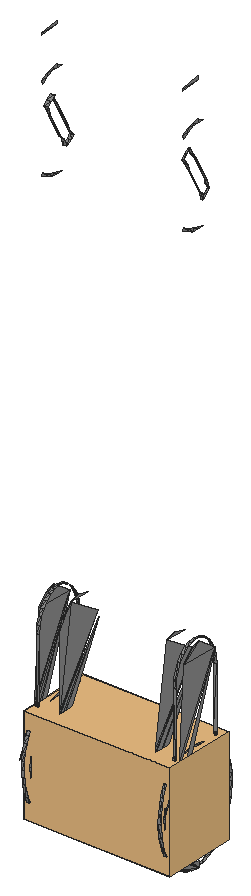
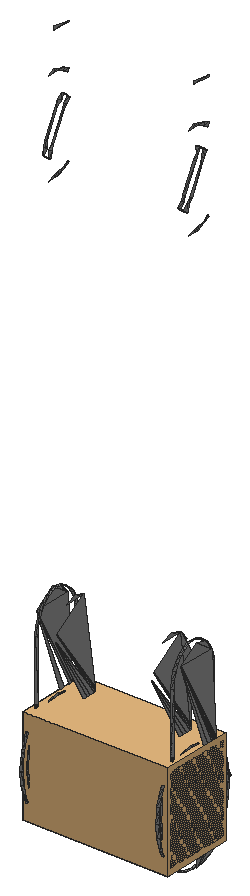
# SketchUp Ruby script. Lengths in inches.
U = 1.inch
M = Sketchup.active_model
def pt(a) = Geom::Point3d.new(a.map { |v| v * U })
def face(e, loops, mat)
  f = e.add_face(loops[0].map { |a| pt(a) })
  loops[1..].each { |l| e.add_face(l.map { |a| pt(a) }).erase! }
  f.material = f.back_material = mat if mat
  f
end
# faces: each face lists its corners as indices into pts; further lists are holes
def faces(e, pts, list, mat = nil) = list.each { |f| face(e, (f[0].is_a?(Array) ? f : [f]).map { |l| l.map { |i| pts[i] } }, mat) }
# xy, xz, yz: faces in a plane at the given z, y or x. An outline is a flat list of corners, or four numbers for a rectangle; further outlines are holes
def ring(l) = l.size == 4 ? [[l[0], l[1]], [l[2], l[1]], [l[2], l[3]], [l[0], l[3]]] : l.each_slice(2).to_a
def flat(e, list, mat, &to3) = list.each { |f| face(e, (f[0].is_a?(Array) ? f : [f]).map { |l| ring(l).map { |u, v| to3.(u, v) } }, mat) }
def xy(e, z, list, mat = nil) = flat(e, list, mat) { |x, y| [x, y, z] }
def xz(e, y, list, mat = nil) = flat(e, list, mat) { |x, z| [x, y, z] }
def yz(e, x, list, mat = nil) = flat(e, list, mat) { |y, z| [x, y, z] }
def lines(e, pts, list) = list.each { |a, b| e.add_line(pt(pts[a]), pt(pts[b])) }
# prism: a flat outline (further loops are holes) pulled along v
def prism(e, loops, v, mat = nil)
  f = face(e, loops, mat); d = Geom::Vector3d.new(v.map { |x| x * U })
  f.pushpull(f.normal.samedirection?(d) ? d.length : -d.length)
end
def box(e, o, s, mat = nil) = prism(e, [[o, [o[0] + s[0], o[1], o[2]], [o[0] + s[0], o[1] + s[1], o[2]], [o[0], o[1] + s[1], o[2]]]], [0, 0, s[2]], mat)
def at(x, y, z, deg = 0) = Geom::Transformation.translation(pt([x, y, z])) * Geom::Transformation.rotation(ORIGIN, Z_AXIS, deg.degrees)
def axes(o, x, y, z) = Geom::Transformation.new([*x, 0, *y, 0, *z, 0, *pt(o).to_a, 1])
def part(name) = M.definitions.add(name)
# library, detail: a bought-in or finely detailed component or shape, given as its bounding box
def library(name, o, s) = part(name).tap { |d| box(d.entities, o, s) }
def detail(e, o, s) = box(e.add_group.entities, o, s)
def put(e, d, t, mat = nil) = e.add_instance(d, t).tap { |i| i.material = mat if mat }
def group(e, t, mat = nil) = e.add_group.tap { |g| g.transformation = t; g.material = mat if mat }.entities
root = M.entities
M.materials.add("Material \#1").color = [140, 140, 140]
c1 = library("3DGeom~12_Defintion",[-95.68,-755.75,-830.03],[191.36,191.37,1000])
c2 = part("3DGeom~10_Defintion")
yz(c2.entities,-68.96,[[-797.08,-844.83,-797.08,-827.59,-922.41,-827.59],[-922.41,-844.83,-797.08,-844.83,-922.41,-827.59]],"Material \#1")
yz(c2.entities,68.97,[[-922.41,-844.83,-797.08,-827.59,-797.08,-844.83],[-922.41,-844.83,-922.41,-827.59,-797.08,-827.59],[-797.08,137.93,-922.41,155.17,-797.08,155.17],[-922.41,137.93,-922.41,155.17,-797.08,137.93]],"Material \#1")
p = [[-15.8,-989.55,-844.83],[-15.8,-989.55,-827.59],[0,-991.38,-827.59],[0,-991.38,-844.83],[15.8,-989.55,-827.59],[15.8,-989.55,-844.83],
  [-30.32,-984.36,-844.83],[-30.32,-984.36,-827.59],[30.31,-984.36,-827.59],[30.31,-984.36,-844.83],[-43.12,-976.21,-844.83],[-43.12,-976.21,-827.59],
  [43.12,-976.21,-827.59],[43.12,-976.21,-844.83],[-53.81,-965.53,-844.83],[-53.81,-965.53,-827.59],[53.8,-965.53,-827.59],[53.8,-965.53,-844.83],
  [-61.95,-952.73,-844.83],[-61.95,-952.73,-827.59],[53.8,-965.53,-827.59],[61.95,-952.73,-827.59],[61.95,-952.73,-844.83],[-67.15,-938.21,-844.83],
  [-67.15,-938.21,-827.59],[67.14,-938.21,-827.59],[67.14,-938.21,-844.83],[-68.96,-922.41,-844.83],[-68.96,-922.41,-827.59],[67.14,-938.21,-827.59],
  [68.97,-922.41,-827.59],[68.97,-922.41,-844.83],[-69.1,-794.86,-844.83],[-69.1,-794.86,-827.59],[-68.96,-797.08,-827.59],[-68.96,-797.08,-844.83],
  [68.97,-797.08,-844.83],[68.97,-797.08,-827.59],[69.11,-794.71,-827.59],[69.11,-794.71,-844.83],[-69.48,-792.73,-844.83],[-69.48,-792.73,-827.59],
  [69.53,-792.51,-827.59],[69.53,-792.51,-844.83],[-70.14,-790.6875,-844.83],[-70.14,-790.6875,-827.59],[70.24,-790.48,-827.59],[70.24,-790.48,-844.83],
  [-71.08,-788.73,-844.83],[-71.08,-788.73,-827.59],[71.22,-788.57,-827.59],[71.22,-788.57,-844.83],[-72.32,-786.86,-844.83],[-72.32,-786.86,-827.59],
  [72.47,-786.78,-827.59],[72.47,-786.78,-844.83],[-73.8,-785.17,-844.83],[-73.8,-785.17,-827.59],[74,-785.04,-827.59],[74,-785.04,-844.83],
  [-75.96,-783.21,-844.83],[-75.96,-783.21,-827.59],[74,-785.04,-827.59],[75.76,-783.39,-827.59],[75.76,-783.39,-844.83],[86.625,-772.95,-827.59],
  [86.61,-772.96,-844.83],[-86.89,-773.25,-844.83],[-86.89,-773.25,-827.59],[-75.96,-783.21,-844.83],[-96.66,-761.8,-844.83],[-96.66,-761.8,-827.59],
  [86.625,-772.95,-827.59],[86.63,-772.94,-844.83],[86.61,-772.96,-844.83],[86.625,-772.95,-827.59],[86.62,-772.95,-827.59],[86.62,-772.95,-827.59],
  [96.31,-761.375,-827.59],[96.31,-761.375,-844.83],[86.63,-772.94,-844.83],[86.625,-772.95,-827.59],[86.62,-772.95,-827.59],[-104.96,-749.18,-844.83],
  [-104.96,-749.18,-827.59],[-96.66,-761.8,-827.59],[-96.66,-761.8,-844.83],[96.31,-761.375,-827.59],[104.62,-748.77,-827.59],[104.62,-748.77,-844.83],
  [-111.64,-735.52,-844.83],[-111.64,-735.52,-827.59],[111.39,-735.21,-827.59],[111.39,-735.21,-844.83],[-116.49,-721.23,-844.83],[-116.49,-721.23,-827.59],
  [116.4375,-720.78,-827.59],[116.4375,-720.78,-844.83],[-119.64,-705.62,-844.83],[-119.64,-705.62,-827.59],[119.6,-705.57,-827.59],[119.6,-705.57,-844.83],
  [-120.6875,-689.65,-844.83],[-120.6875,-689.65,-827.59],[120.69,-689.65,-827.59],[120.69,-689.65,-844.83],[-117.5,-662,-844.83],[-117.5,-662,-827.59],
  [117.5,-662,-827.59],[117.5,-662,-844.83],[-108.41,-636.61,-844.83],[-108.41,-636.61,-827.59],[117.5,-662,-844.83],[108.41,-636.61,-827.59],
  [108.41,-636.61,-844.83],[-93.91,-613.95,-844.83],[-93.91,-613.95,-827.59],[-108.41,-636.61,-827.59],[108.41,-636.61,-844.83],[94.16,-614.19,-827.59],
  [94.16,-614.19,-844.83],[94.16,-614.19,-827.59],[75.46,-595.5,-827.59],[75.46,-595.5,-844.83],[-75.46,-595.5,-844.83],[-75.46,-595.5,-827.59],
  [-93.91,-613.95,-827.59],[-93.91,-613.95,-827.59],[-93.91,-613.95,-844.83],[-53.05,-581.24,-844.83],[-53.05,-581.24,-827.59],[-75.46,-595.5,-827.59],
  [-75.46,-595.5,-844.83],[53.05,-581.24,-827.59],[53.05,-581.24,-844.83],[-27.65,-572.16,-844.83],[-27.65,-572.16,-827.59],[-53.05,-581.24,-827.59],
  [-53.05,-581.24,-844.83],[27.66,-572.16,-827.59],[27.66,-572.16,-844.83],[0,-568.97,-844.83],[0,-568.97,-827.59],[-27.65,-572.16,-827.59],
  [-27.65,-572.16,-844.83],[0,-568.97,-844.83],[-15.8,-989.55,155.17],[0,-991.38,155.17],[0,-991.38,137.93],[-15.8,-989.55,137.93],
  [15.8,-989.55,155.17],[15.8,-989.55,137.93],[-30.32,-984.36,155.17],[-30.32,-984.36,137.93],[30.31,-984.36,155.17],[30.31,-984.36,137.93],
  [-43.125,-976.22,155.17],[-43.125,-976.22,137.93],[43.12,-976.22,155.17],[43.12,-976.22,137.93],[-53.81,-965.53,155.17],[-53.81,-965.53,137.93],
  [53.8,-965.53,155.17],[53.8,-965.53,137.93],[-61.96,-952.73,155.17],[-61.95,-952.73,137.93],[61.95,-952.73,155.17],[61.95,-952.73,137.93],
  [53.8,-965.53,137.93],[-67.15,-938.21,155.17],[-67.15,-938.21,137.93],[67.14,-938.21,155.17],[67.14,-938.21,137.93],[-68.96,-922.41,155.17],
  [-68.96,-922.41,137.93],[68.97,-922.41,155.17],[68.97,-922.41,137.93],[67.14,-938.21,137.93],[-68.97,-797.08,155.17],[-68.97,-797.08,137.93],
  [-69.1,-794.86,155.17],[-69.1,-794.86,137.93],[68.97,-797.08,155.17],[69.11,-794.71,155.17],[69.11,-794.71,137.93],[68.97,-797.08,137.93],
  [-69.48,-792.73,155.17],[-69.48,-792.73,137.93],[69.53,-792.51,155.17],[69.53,-792.51,137.93],[-70.14,-790.6875,155.17],[-70.14,-790.6875,137.93],
  [70.24,-790.48,155.17],[70.24,-790.48,137.93],[-71.08,-788.73,155.17],[-71.08,-788.73,137.93],[71.22,-788.57,155.17],[71.22,-788.57,137.93],
  [-72.32,-786.86,155.17],[-72.32,-786.86,137.93],[72.47,-786.78,155.17],[72.47,-786.78,137.93],[-73.8,-785.17,155.17],[-73.8,-785.17,137.93],
  [74,-785.04,155.17],[74,-785.04,137.93],[-75.96,-783.21,155.17],[-75.96,-783.21,137.93],[75.76,-783.39,155.17],[75.76,-783.39,137.93],
  [74,-785.04,137.93],[86.61,-772.96,155.17],[86.625,-772.95,137.93],[-86.88,-773.25,155.17],[-75.96,-783.21,155.17],[-86.88,-773.25,137.93],
  [-96.66,-761.8,155.17],[-96.66,-761.8,137.93],[86.63,-772.94,155.17],[86.625,-772.95,137.93],[86.61,-772.96,155.17],[86.62,-772.95,137.93],
  [86.625,-772.95,137.93],[96.31,-761.375,155.17],[96.31,-761.375,137.93],[86.62,-772.95,137.93],[86.63,-772.94,155.17],[86.62,-772.95,137.93],
  [86.625,-772.95,137.93],[-104.96,-749.18,155.17],[-96.66,-761.8,155.17],[-96.66,-761.8,137.93],[-104.96,-749.18,137.93],[104.62,-748.77,155.17],
  [104.62,-748.77,137.93],[96.31,-761.375,137.93],[-111.64,-735.52,155.17],[-111.64,-735.52,137.93],[111.39,-735.21,155.17],[111.39,-735.21,137.93],
  [-116.49,-721.23,155.17],[-116.49,-721.23,137.93],[116.4375,-720.78,155.17],[116.4375,-720.78,137.93],[-119.64,-705.62,155.17],[-119.64,-705.62,137.93],
  [119.6,-705.57,155.17],[119.6,-705.57,137.93],[-120.6875,-689.65,155.17],[-120.6875,-689.65,137.93],[120.69,-689.65,155.17],[120.69,-689.65,137.93],
  [-117.5,-662,155.17],[-117.5,-662,137.93],[117.5,-662,155.17],[117.5,-662,137.93],[-108.41,-636.61,155.17],[-108.41,-636.61,137.93],
  [117.5,-662,155.17],[108.41,-636.61,155.17],[108.41,-636.61,137.93],[-93.91,-613.95,155.17],[-108.41,-636.61,137.93],[-93.91,-613.95,137.93],
  [108.41,-636.61,155.17],[94.16,-614.19,155.17],[94.16,-614.19,137.93],[75.46,-595.5,155.17],[75.46,-595.5,137.93],[94.16,-614.19,137.93],
  [-75.46,-595.5,155.17],[-93.91,-613.95,155.17],[-93.91,-613.95,137.93],[-75.46,-595.5,137.93],[-53.05,-581.24,155.17],[-75.46,-595.5,155.17],
  [-75.46,-595.5,137.93],[-53.05,-581.24,137.93],[53.05,-581.24,155.17],[53.05,-581.24,137.93],[-27.65,-572.16,155.17],[-53.05,-581.24,155.17],
  [-53.05,-581.24,137.93],[-27.65,-572.16,137.93],[27.65,-572.16,155.17],[27.65,-572.16,137.93],[0,-568.97,155.17],[-27.65,-572.16,155.17],
  [-27.65,-572.16,137.93],[0,-568.97,137.93],[0,-568.97,155.17]]
faces(c2.entities,p,[[0,1,2],[2,3,0],[3,2,4],[4,5,3],[6,7,1],[1,0,6],[5,4,8],[8,9,5],
  [10,11,7],[7,6,10],[9,8,12],[12,13,9],[14,15,11],[11,10,14],[13,12,16],[16,17,13],
  [18,19,15],[15,14,18],[17,20,21],[21,22,17],[23,24,19],[19,18,23],[22,21,25],[25,26,22],
  [27,28,24],[24,23,27],[26,29,30],[30,31,26],[32,33,34],[34,35,32],[36,37,38],[38,39,36],
  [40,41,33],[33,32,40],[39,38,42],[42,43,39],[44,45,41],[41,40,44],[43,42,46],[46,47,43],
  [48,49,45],[45,44,48],[47,46,50],[50,51,47],[52,53,49],[49,48,52],[51,50,54],[54,55,51],
  [56,57,53],[53,52,56],[55,54,58],[58,59,55],[60,61,57],[57,56,60],[59,62,63],[63,64,59],
  [64,63,65],[65,66,64],[67,68,61],[61,69,67],[70,71,68],[68,67,70],[72,73,66],[74,75,76],
  [73,77,78],[78,79,73],[80,81,82],[83,84,85],[85,86,83],[79,87,88],[88,89,79],[90,91,84],
  [84,83,90],[89,88,92],[92,93,89],[94,95,91],[91,90,94],[93,92,96],[96,97,93],[98,99,95],
  [95,94,98],[97,96,100],[100,101,97],[102,103,99],[99,98,102],[101,100,104],[104,105,101],[106,107,103],
  [103,102,106],[105,104,108],[108,109,105],[110,111,107],[107,106,110],[112,108,113],[113,114,112],[115,116,117],
  [117,110,115],[118,113,119],[119,120,118],[120,121,122],[122,123,120],[124,125,126],[127,128,124],[129,130,131],
  [131,132,129],[123,122,133],[133,134,123],[135,136,137],[137,138,135],[134,133,139],[139,140,134],[141,142,143],
  [143,144,141],[140,139,142],[142,145,140],[146,147,148],[148,149,146],[147,150,151],[151,148,147],[152,146,149],
  [149,153,152],[150,154,155],[155,151,150],[156,152,153],[153,157,156],[154,158,159],[159,155,154],[160,156,157],
  [157,161,160],[158,162,163],[163,159,158],[164,160,161],[161,165,164],[162,166,167],[167,168,162],[169,164,165],
  [165,170,169],[166,171,172],[172,167,166],[173,169,170],[170,174,173],[171,175,176],[176,177,171],[178,173,174],
  [174,179,178],[180,178,179],[179,181,180],[182,183,184],[184,185,182],[186,180,181],[181,187,186],[183,188,189],
  [189,184,183],[190,186,187],[187,191,190],[188,192,193],[193,189,188],[194,190,191],[191,195,194],[192,196,197],
  [197,193,192],[198,194,195],[195,199,198],[196,200,201],[201,197,196],[202,198,199],[199,203,202],[200,204,205],
  [205,201,200],[206,202,203],[203,207,206],[204,208,209],[209,210,204],[208,211,212],[212,209,208],[213,214,207],
  [207,215,213],[216,213,215],[215,217,216],[211,218,219],[220,221,222],[218,223,224],[224,225,218],[226,227,228],
  [229,230,231],[231,232,229],[223,233,234],[234,235,223],[236,229,232],[232,237,236],[233,238,239],[239,234,233],
  [240,236,237],[237,241,240],[238,242,243],[243,239,238],[244,240,241],[241,245,244],[242,246,247],[247,243,242],
  [248,244,245],[245,249,248],[246,250,251],[251,247,246],[252,248,249],[249,253,252],[250,254,255],[255,251,250],
  [256,252,253],[253,257,256],[258,259,260],[260,255,258],[261,256,262],[262,263,261],[264,265,266],[266,260,264],
  [265,267,268],[268,269,265],[270,271,272],[272,273,270],[274,275,276],[276,277,274],[267,278,279],[279,268,267],
  [280,281,282],[282,283,280],[278,284,285],[285,279,278],[286,287,288],[288,289,286],[284,290,289],[289,285,284]],"Material \#1")
c3 = library("3DGeom~13_Defintion",[-84.91,-744.98,-830.03],[169.82,169.83,1000])
xy(root,58.25,[[265.622,260.488,265.755,260.488,265.622,260.542],[265.755,260.488,265.755,260.542,265.622,260.542],[266.352,260.488,266.484,260.488,266.484,260.542],[266.352,260.488,266.484,260.542,266.352,260.542]],"Material \#1")
xy(root,58.647,[[265.622,260.504,265.622,260.537,265.755,260.537],[265.622,260.504,265.755,260.537,265.755,260.504],[266.352,260.504,266.352,260.537,266.484,260.504],[266.484,260.504,266.352,260.537,266.484,260.537]],"Material \#1")
xz(root,260.488,[[265.622,58.25,265.755,58.315,265.755,58.25],[266.352,58.25,266.352,58.315,266.484,58.25]],"Material \#1")
xz(root,260.493,[[265.622,58.538,265.755,58.575,265.755,58.538],[266.352,58.538,266.352,58.575,266.484,58.538]],"Material \#1")
yz(root,265.627,[[260.515,58.112,260.316,58.238,260.416,58.182],[260.515,58.112,260.403,58.146,260.316,58.238],[260.515,58.112,260.456,58.121,260.403,58.146],[260.515,58.112,260.416,58.182,260.463,58.159],[260.515,58.112,260.463,58.159,260.515,58.151],
  [260.262,58.493,260.367,58.728,260.626,59.235],[260.339,58.634,260.626,59.235,260.374,58.68],[260.374,58.68,260.626,59.235,260.416,58.716],[260.416,58.716,260.626,59.235,260.463,58.738],[260.367,58.728,260.369,58.735,260.626,59.235],
  [260.369,58.735,260.371,58.742,260.626,59.235],[260.371,58.742,260.372,58.75,260.626,59.235],[260.372,58.75,260.404,59.235,260.626,59.235],[260.404,59.235,260.452,59.286,260.515,59.306],[260.404,59.235,260.515,59.306,260.626,59.235],
  [260.452,59.286,260.482,59.301,260.515,59.306]],"Material \#1")
yz(root,265.641,[[260.515,61.479,260.476,61.484,260.478,61.499],[260.515,61.479,260.478,61.499,260.515,61.494],[260.515,61.479,260.515,61.494,260.554,61.484],[260.476,61.484,260.439,61.498,260.443,61.511],[260.476,61.484,260.443,61.511,260.478,61.499],
  [260.439,61.498,260.405,61.519,260.41,61.532],[260.439,61.498,260.41,61.532,260.443,61.511],[260.41,62.003,260.405,62.016,260.443,62.023],[260.405,62.016,260.439,62.037,260.443,62.023],[260.443,62.023,260.439,62.037,260.478,62.036],
  [260.478,62.036,260.439,62.037,260.476,62.051],[260.478,62.036,260.476,62.051,260.515,62.04],[260.552,62.036,260.515,62.04,260.515,62.055],[260.515,62.04,260.476,62.051,260.515,62.055],[260.399,62.258,260.397,62.273,260.515,62.272],
  [260.515,62.272,260.397,62.273,260.515,62.287]],"Material \#1")
yz(root,265.655,[[260.515,58.151,260.457,58.162,260.458,58.171],[260.515,58.151,260.458,58.171,260.515,58.161],[260.515,58.151,260.515,58.161,260.573,58.162],[260.515,58.161,260.571,58.171,260.573,58.162],[260.457,58.162,260.402,58.191,260.406,58.2],
  [260.457,58.162,260.406,58.2,260.458,58.171],[260.573,58.162,260.571,58.171,260.627,58.191],[260.571,58.171,260.623,58.2,260.627,58.191],[260.402,58.191,260.356,58.238,260.361,58.246],[260.402,58.191,260.361,58.246,260.406,58.2],
  [260.627,58.191,260.623,58.2,260.674,58.238],[260.623,58.2,260.668,58.246,260.674,58.238],[260.356,58.238,260.32,58.3,260.327,58.305],[260.356,58.238,260.327,58.305,260.361,58.246],[260.674,58.238,260.668,58.246,260.71,58.3],
  [260.668,58.246,260.703,58.305,260.71,58.3],[260.32,58.3,260.297,58.372,260.305,58.374],[260.32,58.3,260.305,58.374,260.327,58.305],[260.71,58.3,260.703,58.305,260.732,58.372],[260.703,58.305,260.725,58.374,260.732,58.372],
  [260.297,58.372,260.29,58.449,260.297,58.449],[260.297,58.372,260.297,58.449,260.305,58.374],[260.732,58.372,260.725,58.374,260.74,58.449],[260.725,58.374,260.732,58.449,260.74,58.449],[260.29,58.449,260.297,58.526,260.305,58.523],
  [260.29,58.449,260.305,58.523,260.297,58.449],[260.732,58.449,260.725,58.523,260.732,58.526],[260.732,58.449,260.732,58.526,260.74,58.449],[260.305,58.523,260.297,58.526,260.327,58.592],[260.725,58.523,260.703,58.592,260.71,58.597],
  [260.725,58.523,260.71,58.597,260.732,58.526],[260.297,58.526,260.32,58.597,260.327,58.592],[260.327,58.592,260.32,58.597,260.361,58.652],[260.703,58.592,260.668,58.652,260.674,58.659],[260.703,58.592,260.674,58.659,260.71,58.597],
  [260.32,58.597,260.356,58.659,260.361,58.652],[260.361,58.652,260.356,58.659,260.406,58.697],[260.668,58.652,260.623,58.697,260.627,58.706],[260.668,58.652,260.627,58.706,260.674,58.659],[260.356,58.659,260.402,58.706,260.406,58.697],
  [260.406,58.697,260.402,58.706,260.458,58.726],[260.623,58.697,260.571,58.726,260.573,58.736],[260.623,58.697,260.573,58.736,260.627,58.706],[260.402,58.706,260.457,58.736,260.458,58.726],[260.458,58.726,260.457,58.736,260.515,58.736],
  [260.571,58.726,260.515,58.736,260.515,58.746],[260.571,58.726,260.515,58.746,260.573,58.736],[260.457,58.736,260.515,58.746,260.515,58.736]],"Material \#1")
yz(root,265.755,[[260.488,58.25,260.488,58.315,260.542,58.25],[260.542,58.25,260.488,58.315,260.542,58.315],[260.488,58.315,260.495,58.32,260.542,58.315],[260.542,58.315,260.495,58.32,260.536,58.32],[260.495,58.32,260.495,58.33,260.536,58.32],
  [260.536,58.32,260.495,58.33,260.536,58.33],[260.495,58.33,260.488,58.335,260.536,58.33],[260.536,58.33,260.488,58.335,260.542,58.335],[260.488,58.335,260.488,58.399,260.542,58.335],[260.542,58.335,260.488,58.399,260.542,58.399],
  [260.488,58.399,260.493,58.419,260.542,58.399],[260.542,58.399,260.493,58.419,260.537,58.419],[260.493,58.419,260.485,58.447,260.537,58.419],[260.537,58.419,260.485,58.447,260.545,58.447],[260.485,58.447,260.485,58.475,260.545,58.447],
  [260.545,58.447,260.485,58.475,260.545,58.475],[260.485,58.475,260.493,58.503,260.545,58.475],[260.545,58.475,260.493,58.503,260.537,58.503],[260.493,58.503,260.493,58.538,260.537,58.503],[260.537,58.503,260.493,58.538,260.537,58.538],
  [260.493,58.538,260.493,58.575,260.537,58.538],[260.537,58.538,260.493,58.575,260.526,58.575],[260.493,58.575,260.488,58.585,260.526,58.575],[260.526,58.575,260.488,58.585,260.532,58.585],[260.488,58.585,260.488,58.607,260.532,58.585],
  [260.532,58.585,260.488,58.607,260.532,58.607],[260.488,58.607,260.493,58.617,260.532,58.607],[260.532,58.607,260.493,58.617,260.526,58.617],[260.493,58.617,260.504,58.647,260.526,58.617],[260.526,58.617,260.504,58.647,260.537,58.647]],"Material \#1")
yz(root,265.769,[[260.515,58.112,260.416,58.182,260.316,58.238],[260.515,58.112,260.403,58.146,260.456,58.121],[260.515,58.112,260.463,58.159,260.416,58.182],[260.515,58.112,260.515,58.151,260.463,58.159],[260.339,58.634,260.374,58.68,260.657,59.117],
  [260.339,58.634,260.657,59.117,260.367,58.728],[260.374,58.68,260.416,58.716,260.657,59.117],[260.416,58.716,260.463,58.738,260.657,59.117],[260.367,58.728,260.653,59.16,260.369,58.735],[260.369,58.735,260.653,59.16,260.371,58.742],
  [260.371,58.742,260.653,59.16,260.372,58.75],[260.372,58.75,260.653,59.16,260.372,58.757],[260.372,58.757,260.452,59.286,260.376,59.16],[260.372,58.757,260.653,59.16,260.452,59.286],[260.404,59.235,260.452,59.286,260.426,59.264],
  [260.452,59.286,260.515,59.306,260.482,59.301],[260.452,59.286,260.577,59.286,260.515,59.306]],"Material \#1")
yz(root,266.338,[[260.515,58.112,260.316,58.238,260.416,58.182],[260.515,58.112,260.403,58.146,260.316,58.238],[260.515,58.112,260.456,58.121,260.403,58.146],[260.515,58.112,260.416,58.182,260.463,58.159],[260.515,58.112,260.463,58.159,260.515,58.151],
  [260.339,58.634,260.367,58.728,260.657,59.117],[260.339,58.634,260.657,59.117,260.374,58.68],[260.374,58.68,260.657,59.117,260.416,58.716],[260.416,58.716,260.657,59.117,260.463,58.738],[260.367,58.728,260.369,58.735,260.653,59.16],
  [260.369,58.735,260.371,58.742,260.653,59.16],[260.371,58.742,260.372,58.75,260.653,59.16],[260.372,58.75,260.372,58.757,260.653,59.16],[260.372,58.757,260.452,59.286,260.653,59.16],[260.452,59.286,260.482,59.301,260.515,59.306],
  [260.452,59.286,260.515,59.306,260.577,59.286]],"Material \#1")
yz(root,266.352,[[260.488,58.25,260.542,58.25,260.488,58.315],[260.542,58.25,260.542,58.315,260.488,58.315],[260.488,58.315,260.542,58.315,260.495,58.32],[260.542,58.315,260.536,58.32,260.495,58.32],[260.495,58.32,260.536,58.32,260.495,58.33],
  [260.536,58.32,260.536,58.33,260.495,58.33],[260.495,58.33,260.536,58.33,260.488,58.335],[260.536,58.33,260.542,58.335,260.488,58.335],[260.488,58.335,260.542,58.335,260.488,58.399],[260.542,58.335,260.542,58.399,260.488,58.399],
  [260.488,58.399,260.542,58.399,260.493,58.419],[260.542,58.399,260.537,58.419,260.493,58.419],[260.493,58.419,260.537,58.419,260.485,58.447],[260.537,58.419,260.545,58.447,260.485,58.447],[260.485,58.447,260.545,58.447,260.485,58.475],
  [260.545,58.447,260.545,58.475,260.485,58.475],[260.485,58.475,260.545,58.475,260.493,58.503],[260.545,58.475,260.537,58.503,260.493,58.503],[260.493,58.503,260.537,58.503,260.493,58.538],[260.537,58.503,260.537,58.538,260.493,58.538],
  [260.493,58.538,260.537,58.538,260.493,58.575],[260.537,58.538,260.526,58.575,260.493,58.575],[260.493,58.575,260.526,58.575,260.488,58.585],[260.526,58.575,260.532,58.585,260.488,58.585],[260.488,58.585,260.532,58.585,260.488,58.607],
  [260.532,58.585,260.532,58.607,260.488,58.607],[260.488,58.607,260.532,58.607,260.493,58.617],[260.532,58.607,260.526,58.617,260.493,58.617],[260.493,58.617,260.526,58.617,260.504,58.647],[260.526,58.617,260.537,58.647,260.504,58.647]],"Material \#1")
yz(root,266.451,[[260.515,58.151,260.458,58.171,260.457,58.162],[260.515,58.151,260.515,58.161,260.458,58.171],[260.515,58.151,260.573,58.162,260.515,58.161],[260.515,58.161,260.573,58.162,260.571,58.171],[260.457,58.162,260.406,58.2,260.402,58.191],
  [260.457,58.162,260.458,58.171,260.406,58.2],[260.573,58.162,260.627,58.191,260.571,58.171],[260.571,58.171,260.627,58.191,260.623,58.2],[260.402,58.191,260.361,58.246,260.356,58.238],[260.402,58.191,260.406,58.2,260.361,58.246],
  [260.627,58.191,260.674,58.238,260.623,58.2],[260.623,58.2,260.674,58.238,260.668,58.246],[260.356,58.238,260.326,58.305,260.32,58.3],[260.356,58.238,260.361,58.246,260.326,58.305],[260.674,58.238,260.71,58.3,260.668,58.246],
  [260.668,58.246,260.71,58.3,260.703,58.305],[260.32,58.3,260.305,58.374,260.297,58.372],[260.32,58.3,260.326,58.305,260.305,58.374],[260.71,58.3,260.732,58.372,260.703,58.305],[260.703,58.305,260.732,58.372,260.725,58.374],
  [260.297,58.372,260.297,58.449,260.29,58.449],[260.297,58.372,260.305,58.374,260.297,58.449],[260.732,58.372,260.74,58.449,260.725,58.374],[260.725,58.374,260.74,58.449,260.732,58.449],[260.29,58.449,260.297,58.449,260.305,58.523],
  [260.29,58.449,260.305,58.523,260.297,58.526],[260.732,58.449,260.732,58.526,260.725,58.523],[260.732,58.449,260.74,58.449,260.732,58.526],[260.305,58.523,260.326,58.592,260.297,58.526],[260.725,58.523,260.71,58.597,260.703,58.592],
  [260.725,58.523,260.732,58.526,260.71,58.597],[260.297,58.526,260.326,58.592,260.32,58.597],[260.326,58.592,260.361,58.652,260.32,58.597],[260.703,58.592,260.674,58.659,260.668,58.652],[260.703,58.592,260.71,58.597,260.674,58.659],
  [260.32,58.597,260.361,58.652,260.356,58.659],[260.361,58.652,260.406,58.697,260.356,58.659],[260.668,58.652,260.627,58.706,260.623,58.697],[260.668,58.652,260.674,58.659,260.627,58.706],[260.356,58.659,260.406,58.697,260.402,58.706],
  [260.406,58.697,260.458,58.726,260.402,58.706],[260.623,58.697,260.573,58.736,260.571,58.726],[260.623,58.697,260.627,58.706,260.573,58.736],[260.402,58.706,260.458,58.726,260.457,58.736],[260.458,58.726,260.515,58.736,260.457,58.736],
  [260.571,58.726,260.515,58.746,260.515,58.736],[260.571,58.726,260.573,58.736,260.515,58.746],[260.457,58.736,260.515,58.736,260.515,58.746]],"Material \#1")
yz(root,266.465,[[260.515,61.479,260.478,61.499,260.476,61.484],[260.515,61.479,260.515,61.494,260.478,61.499],[260.515,61.479,260.554,61.484,260.515,61.494],[260.476,61.484,260.443,61.511,260.439,61.498],[260.476,61.484,260.478,61.499,260.443,61.511],
  [260.439,61.498,260.41,61.532,260.405,61.519],[260.439,61.498,260.443,61.511,260.41,61.532],[260.41,62.003,260.443,62.023,260.405,62.016],[260.405,62.016,260.443,62.023,260.439,62.037],[260.443,62.023,260.478,62.036,260.439,62.037],
  [260.478,62.036,260.476,62.051,260.439,62.037],[260.478,62.036,260.515,62.04,260.476,62.051],[260.552,62.036,260.515,62.055,260.515,62.04],[260.515,62.04,260.515,62.055,260.476,62.051],[260.399,62.258,260.515,62.272,260.397,62.273],
  [260.515,62.272,260.515,62.287,260.397,62.273]],"Material \#1")
yz(root,266.48,[[260.515,58.112,260.316,58.238,260.403,58.146],[260.515,58.112,260.416,58.182,260.316,58.238],[260.515,58.112,260.403,58.146,260.456,58.121],[260.515,58.112,260.463,58.159,260.416,58.182],[260.515,58.112,260.515,58.151,260.463,58.159],
  [260.262,58.493,260.626,59.235,260.367,58.728],[260.416,58.716,260.463,58.738,260.626,59.235],[260.372,58.75,260.626,59.235,260.404,59.235],[260.404,59.235,260.452,59.286,260.426,59.264],[260.404,59.235,260.515,59.306,260.452,59.286],
  [260.404,59.235,260.626,59.235,260.515,59.306],[260.452,59.286,260.515,59.306,260.482,59.301]],"Material \#1")
yz(root,266.484,[[260.515,58.184,260.465,58.202,260.463,58.193],[260.515,58.184,260.515,58.194,260.465,58.202],[260.515,58.184,260.567,58.193,260.515,58.194],[260.463,58.193,260.418,58.228,260.415,58.219],[260.463,58.193,260.465,58.202,260.418,58.228],
  [260.567,58.193,260.565,58.202,260.515,58.194],[260.567,58.193,260.615,58.219,260.565,58.202],[260.565,58.202,260.615,58.219,260.611,58.228],[260.415,58.219,260.378,58.268,260.373,58.261],[260.415,58.219,260.418,58.228,260.378,58.268],
  [260.615,58.219,260.657,58.261,260.611,58.228],[260.611,58.228,260.657,58.261,260.651,58.268],[260.373,58.261,260.348,58.321,260.341,58.316],[260.373,58.261,260.378,58.268,260.348,58.321],[260.657,58.261,260.688,58.316,260.651,58.268],
  [260.651,58.268,260.688,58.316,260.682,58.321],[260.341,58.316,260.328,58.383,260.321,58.38],[260.341,58.316,260.348,58.321,260.328,58.383],[260.688,58.316,260.708,58.38,260.682,58.321],[260.682,58.321,260.708,58.38,260.701,58.383],
  [260.321,58.38,260.322,58.449,260.314,58.449],[260.321,58.38,260.328,58.383,260.322,58.449],[260.708,58.38,260.715,58.449,260.701,58.383],[260.701,58.383,260.715,58.449,260.708,58.449],[260.314,58.449,260.322,58.449,260.328,58.515],
  [260.314,58.449,260.328,58.515,260.321,58.517],[260.708,58.449,260.708,58.517,260.701,58.515],[260.708,58.449,260.715,58.449,260.708,58.517],[260.328,58.515,260.348,58.576,260.321,58.517],[260.701,58.515,260.688,58.581,260.682,58.576],
  [260.701,58.515,260.708,58.517,260.688,58.581],[260.321,58.517,260.348,58.576,260.341,58.581],[260.348,58.576,260.378,58.629,260.341,58.581],[260.682,58.576,260.657,58.636,260.651,58.629],[260.682,58.576,260.688,58.581,260.657,58.636],
  [260.341,58.581,260.378,58.629,260.373,58.636],[260.378,58.629,260.418,58.669,260.373,58.636],[260.651,58.629,260.615,58.678,260.611,58.669],[260.651,58.629,260.657,58.636,260.615,58.678],[260.373,58.636,260.418,58.669,260.415,58.678],
  [260.418,58.669,260.465,58.695,260.415,58.678],[260.611,58.669,260.567,58.704,260.565,58.695],[260.611,58.669,260.615,58.678,260.567,58.704],[260.415,58.678,260.465,58.695,260.463,58.704],[260.465,58.695,260.515,58.703,260.463,58.704],
  [260.565,58.695,260.515,58.713,260.515,58.703],[260.565,58.695,260.567,58.704,260.515,58.713],[260.515,58.703,260.515,58.713,260.463,58.704]],"Material \#1")
p = [[265.755,260.488,58.399],[265.755,260.488,58.335],[265.622,260.49,58.329],[265.622,260.488,58.25],[265.622,260.49,58.329],[265.755,260.488,58.315],
  [265.622,260.49,58.329],[265.622,260.488,58.395],[265.755,260.488,58.399],[265.622,260.539,58.323],[265.755,260.536,58.33],[265.755,260.542,58.335],
  [265.622,260.49,58.329],[265.755,260.495,58.33],[265.755,260.495,58.32],[265.622,260.49,58.329],[265.755,260.488,58.315],[265.622,260.49,58.329],
  [265.755,260.488,58.335],[265.622,260.539,58.323],[265.755,260.542,58.315],[265.755,260.536,58.32],[265.622,260.539,58.323],[266.484,260.49,58.329],
  [266.352,260.488,58.335],[266.352,260.488,58.399],[266.352,260.488,58.315],[266.484,260.49,58.329],[266.484,260.488,58.25],[266.352,260.488,58.399],
  [266.484,260.488,58.395],[266.484,260.49,58.329],[266.484,260.539,58.323],[266.352,260.542,58.335],[266.352,260.536,58.33],[266.484,260.49,58.329],
  [266.352,260.495,58.32],[266.352,260.495,58.33],[266.484,260.49,58.329],[266.352,260.488,58.315],[266.484,260.49,58.329],[266.352,260.488,58.335],
  [266.484,260.539,58.323],[266.352,260.536,58.32],[266.352,260.542,58.315],[266.484,260.539,58.323],[265.755,260.485,58.475],[265.755,260.485,58.447],
  [265.622,260.489,58.433],[265.622,260.489,58.433],[265.622,260.485,58.461],[265.755,260.485,58.475],[265.622,260.491,58.409],[265.622,260.489,58.433],
  [265.755,260.485,58.447],[265.755,260.485,58.447],[265.755,260.493,58.419],[265.622,260.491,58.409],[265.755,260.493,58.419],[265.755,260.488,58.399],
  [265.622,260.488,58.395],[265.622,260.488,58.395],[265.622,260.491,58.409],[265.755,260.493,58.419],[266.484,260.489,58.433],[266.352,260.485,58.447],
  [266.352,260.485,58.475],[266.352,260.485,58.475],[266.484,260.485,58.461],[266.484,260.489,58.433],[266.352,260.485,58.447],[266.484,260.489,58.433],
  [266.484,260.491,58.409],[266.484,260.491,58.409],[266.352,260.493,58.419],[266.352,260.485,58.447],[266.484,260.488,58.395],[266.352,260.488,58.399],
  [266.352,260.493,58.419],[266.352,260.493,58.419],[266.484,260.491,58.409],[266.484,260.488,58.395],[265.755,260.493,58.503],[265.755,260.485,58.475],
  [265.622,260.485,58.461],[265.622,260.485,58.461],[265.622,260.489,58.489],[265.755,260.493,58.503],[265.622,260.489,58.489],[265.622,260.493,58.538],
  [265.755,260.493,58.538],[265.755,260.493,58.538],[265.755,260.493,58.503],[265.622,260.489,58.489],[265.622,260.493,58.538],[265.622,260.49,58.58],
  [265.755,260.493,58.575],[266.484,260.485,58.461],[266.352,260.485,58.475],[266.352,260.493,58.503],[266.352,260.493,58.503],[266.484,260.489,58.489],
  [266.484,260.485,58.461],[266.484,260.489,58.489],[266.352,260.493,58.503],[266.352,260.493,58.538],[266.352,260.493,58.538],[266.484,260.493,58.538],
  [266.484,260.489,58.489],[266.352,260.493,58.575],[266.484,260.49,58.58],[266.484,260.493,58.538],[265.622,260.49,58.58],[265.622,260.49,58.612],
  [265.755,260.488,58.607],[265.755,260.488,58.585],[265.622,260.49,58.58],[265.755,260.488,58.585],[265.755,260.493,58.575],[265.622,260.49,58.612],
  [265.755,260.493,58.617],[265.755,260.488,58.607],[265.622,260.49,58.612],[265.622,260.504,58.647],[265.755,260.504,58.647],[265.755,260.493,58.617],
  [265.622,260.49,58.612],[265.622,260.529,58.58],[265.755,260.526,58.575],[265.755,260.532,58.585],[265.622,260.529,58.612],[265.755,260.532,58.607],
  [265.755,260.526,58.617],[266.484,260.49,58.58],[266.352,260.488,58.585],[266.352,260.488,58.607],[266.484,260.49,58.612],[266.484,260.49,58.58],
  [266.352,260.493,58.575],[266.352,260.488,58.585],[266.484,260.49,58.612],[266.352,260.488,58.607],[266.352,260.493,58.617],[266.484,260.49,58.612],
  [266.352,260.493,58.617],[266.352,260.504,58.647],[266.484,260.504,58.647],[266.484,260.49,58.612],[266.484,260.529,58.58],[266.352,260.532,58.585],
  [266.352,260.526,58.575],[266.484,260.529,58.612],[266.352,260.526,58.617],[266.352,260.532,58.607],[265.644,260.565,61.614],[265.641,260.548,61.645],
  [265.652,260.548,61.645],[265.655,260.565,61.614],[265.64,260.534,61.673],[265.651,260.534,61.673],[266.463,260.565,61.614],[266.451,260.565,61.614],
  [266.454,260.548,61.645],[266.466,260.548,61.645],[266.455,260.534,61.673],[266.467,260.534,61.673],[265.644,260.607,61.653],[265.644,260.588,61.63],
  [265.655,260.588,61.63],[265.655,260.607,61.653],[266.463,260.607,61.653],[266.451,260.607,61.653],[266.451,260.588,61.63],[266.463,260.588,61.63],
  [265.64,260.454,61.823],[265.651,260.454,61.823],[265.64,260.496,61.861],[265.64,260.575,61.712],[265.651,260.575,61.712],[265.651,260.496,61.861],
  [266.455,260.454,61.823],[266.467,260.454,61.823],[266.467,260.496,61.861],[266.455,260.496,61.861],[266.455,260.575,61.712],[266.467,260.575,61.712],
  [265.641,260.59,61.684],[265.652,260.59,61.684],[266.454,260.59,61.684],[266.466,260.59,61.684],[265.641,260.44,61.851],[265.652,260.44,61.851],
  [266.454,260.44,61.851],[266.466,260.44,61.851],[265.644,260.423,61.882],[265.655,260.423,61.882],[265.644,260.442,61.905],[265.655,260.442,61.905],
  [265.644,260.465,61.92],[265.655,260.465,61.92],[266.451,260.423,61.882],[266.463,260.423,61.882],[266.451,260.442,61.905],[266.463,260.442,61.905],
  [266.451,260.465,61.92],[266.463,260.465,61.92],[265.641,260.481,61.889],[265.652,260.481,61.889],[266.454,260.481,61.889],[266.466,260.481,61.889]]
faces(root,p,[[0,1,2],[3,4,5],[6,7,8],[9,10,11],[12,13,14],[15,14,16],[17,18,13],[19,20,21],
  [22,21,10],[23,24,25],[26,27,28],[29,30,31],[32,33,34],[35,36,37],[38,39,36],[40,37,41],
  [42,43,44],[45,34,43],[46,47,48],[49,50,51],[52,53,54],[55,56,57],[58,59,60],[61,62,63],
  [64,65,66],[67,68,69],[70,71,72],[73,74,75],[76,77,78],[79,80,81],[82,83,84],[85,86,87],
  [88,89,90],[91,92,93],[94,95,96],[97,98,99],[100,101,102],[103,104,105],[106,107,108],[109,110,111],
  [112,113,114],[114,115,112],[116,117,118],[119,120,121],[122,123,124],[124,125,126],[127,128,129],[130,131,132],
  [133,134,135],[135,136,133],[137,138,139],[140,141,142],[143,144,145],[145,146,147],[148,149,150],[151,152,153],
  [154,155,156],[156,157,154],[155,158,159],[159,156,155],[160,161,162],[162,163,160],[163,162,164],[164,165,163],
  [166,167,168],[168,169,166],[167,154,157],[157,168,167],[170,171,172],[172,173,170],[173,172,161],[161,160,173],
  [158,174,175],[175,159,158],[176,177,178],[178,179,176],[165,164,180],[180,181,165],[182,183,184],[184,185,182],
  [177,186,187],[187,178,177],[186,166,169],[169,187,186],[185,184,188],[188,189,185],[189,188,171],[171,170,189],
  [174,190,191],[191,175,174],[181,180,192],[192,193,181],[190,194,195],[195,191,190],[194,196,197],[197,195,194],
  [196,198,199],[199,197,196],[193,192,200],[200,201,193],[201,200,202],[202,203,201],[203,202,204],[204,205,203],
  [198,206,207],[207,199,198],[206,176,179],[179,207,206],[205,204,208],[208,209,205],[209,208,183],[183,182,209]],"Material \#1")
put(root,c1,axes([265.77,260.51,56.47],[0,0.00227,0],[0,0,-0.003],[-0.00086,0,0]),"Material \#1")
put(root,c2,axes([265.77,260.51,56.47],[0,0.00217,0],[0,0,-0.00287],[-0.00082,0,0]),"Material \#1")
put(root,c3,axes([265.77,260.51,56.47],[0,0.00227,0],[0,0,-0.003],[-0.00086,0,0]),"Material \#1")
